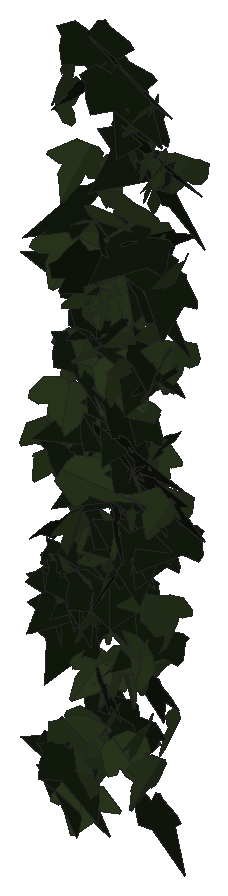
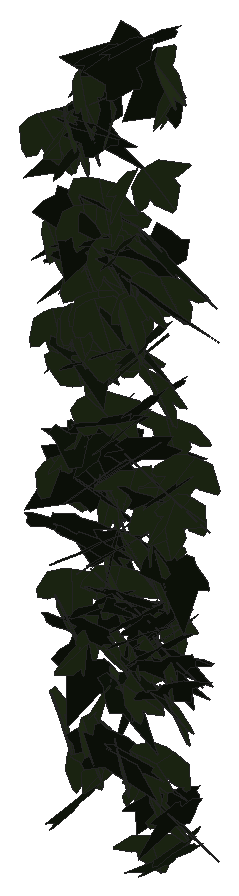
# SketchUp Ruby script. Lengths in inches.
U = 1.inch
M = Sketchup.active_model
def pt(a) = Geom::Point3d.new(a.map { |v| v * U })
def face(e, loops, mat)
  f = e.add_face(loops[0].map { |a| pt(a) })
  loops[1..].each { |l| e.add_face(l.map { |a| pt(a) }).erase! }
  f.material = f.back_material = mat if mat
  f
end
# faces: each face lists its corners as indices into pts; further lists are holes
def faces(e, pts, list, mat = nil) = list.each { |f| face(e, (f[0].is_a?(Array) ? f : [f]).map { |l| l.map { |i| pts[i] } }, mat) }
# xy, xz, yz: faces in a plane at the given z, y or x. An outline is a flat list of corners, or four numbers for a rectangle; further outlines are holes
def ring(l) = l.size == 4 ? [[l[0], l[1]], [l[2], l[1]], [l[2], l[3]], [l[0], l[3]]] : l.each_slice(2).to_a
def flat(e, list, mat, &to3) = list.each { |f| face(e, (f[0].is_a?(Array) ? f : [f]).map { |l| ring(l).map { |u, v| to3.(u, v) } }, mat) }
def xy(e, z, list, mat = nil) = flat(e, list, mat) { |x, y| [x, y, z] }
def xz(e, y, list, mat = nil) = flat(e, list, mat) { |x, z| [x, y, z] }
def yz(e, x, list, mat = nil) = flat(e, list, mat) { |y, z| [x, y, z] }
def lines(e, pts, list) = list.each { |a, b| e.add_line(pt(pts[a]), pt(pts[b])) }
# prism: a flat outline (further loops are holes) pulled along v
def prism(e, loops, v, mat = nil)
  f = face(e, loops, mat); d = Geom::Vector3d.new(v.map { |x| x * U })
  f.pushpull(f.normal.samedirection?(d) ? d.length : -d.length)
end
def box(e, o, s, mat = nil) = prism(e, [[o, [o[0] + s[0], o[1], o[2]], [o[0] + s[0], o[1] + s[1], o[2]], [o[0], o[1] + s[1], o[2]]]], [0, 0, s[2]], mat)
def at(x, y, z, deg = 0) = Geom::Transformation.translation(pt([x, y, z])) * Geom::Transformation.rotation(ORIGIN, Z_AXIS, deg.degrees)
def axes(o, x, y, z) = Geom::Transformation.new([*x, 0, *y, 0, *z, 0, *pt(o).to_a, 1])
def part(name) = M.definitions.add(name)
# library, detail: a bought-in or finely detailed component or shape, given as its bounding box
def library(name, o, s) = part(name).tap { |d| box(d.entities, o, s) }
def detail(e, o, s) = box(e.add_group.entities, o, s)
def put(e, d, t, mat = nil) = e.add_instance(d, t).tap { |i| i.material = mat if mat }
def group(e, t, mat = nil) = e.add_group.tap { |g| g.transformation = t; g.material = mat if mat }.entities
root = M.entities
M.materials.add("1026 AP 7946 SUNNY SIDE UP").color = [254, 231, 186]
M.materials.add("efeu1").color = [18, 25, 13]
M.materials.add("efeu2").color = [43, 57, 29]
c1 = part("ivyleaf_9")
p = [[1.54,2.16,1.25],[1.36,2.04,1.19],[-0.21,0.99,0.68],[-0.71,1.11,0.82],[-0.85,0.86,0.67],[-0.8,0.17,0.21],
  [-0.9,-0.01,0.1],[-0.67,-0.16,-0.02],[-0.08,-0.08,-0.05],[-0.03,-0.6,-0.4],[0.65,-0.88,-0.66],[0.83,-0.6,-0.49],
  [1.29,-0.42,-0.43],[1.8125,-0.07,-0.26],[1.21,0.44,0.15]]
faces(c1.entities,p,[[0,1,2,3,4,5,6,7,8,9,10,11,12,13,14]],"efeu1")
c2 = part("ivyleaf_10")
p = [[0,0.5,-0.03],[-0.0625,2.02,-0.43],[-0.19,2.01,-0.46],[-0.54,1.05,-0.29],[-0.52,0.625,-0.18],[-0.83,0.76,-0.28],
  [-1.16,0.64,-0.33],[-1.15,0.33,-0.24],[-0.77,-0.39,0.02],[-0.3,-0.51,0.16],[0.04,-0.48,0.23],[-0.02,2.01,-0.4375],
  [-0.06,2.01,-0.43],[0.04,-0.49,0.23],[0.67,-0.49,0.14],[1.38,0.36,-0.2],[1.375,0.51,-0.24],[0.81,0.65,-0.19],
  [0.62,0.59,-0.15],[0.6,1.09,-0.28],[0.5,1.23,-0.31]]
faces(c2.entities,p,[[0,1,2,3,4,5,6,7,8,9,10],[11,12,0,13,14,15,16,17,18,19,20]],"efeu2")
put(root,c1,axes([120.77,212.53,268.47],[-0.21091,0.19544,0.14117],[-0.17036,0.08881,-0.24117],[-0.33331,-0.16906,0.03393]),"1026 AP 7946 SUNNY SIDE UP")
put(root,c1,axes([120.59,212.47,271.88],[0.03047,0.27622,-0.0017],[0.01454,-0.00388,-0.28511],[-0.43411,0.01926,-0.00967]),"1026 AP 7946 SUNNY SIDE UP")
put(root,c2,axes([120.49,212.69,270.06],[0.30892,-0.18725,0.0155],[-0.00122,-0.02411,-0.27913],[0.29552,0.19564,-0.01735]),"1026 AP 7946 SUNNY SIDE UP")
put(root,c2,axes([120.4,212.55,272.75],[-0.1299,-0.2003,-0.193],[0.20416,0.14247,-0.21639],[0.37847,-0.1456,0.05049]),"1026 AP 7946 SUNNY SIDE UP")
put(root,c1,axes([120.51,212.87,270.33],[-0.22787,-0.21754,0.05698],[-0.02154,-0.05861,-0.26879],[0.35277,-0.1441,0.02039]),"1026 AP 7946 SUNNY SIDE UP")
put(root,c1,axes([120.47,212.9,270.74],[-0.21926,-0.23495,-0.01553],[0.03784,0.00165,-0.28071],[0.36813,-0.14011,0.0196]),"1026 AP 7946 SUNNY SIDE UP")
put(root,c1,axes([120.75,212.77,276.4],[-0.38855,0.15901,-0.04009],[0.01893,-0.05423,-0.30039],[-0.25705,-0.24435,0.03848]),"1026 AP 7946 SUNNY SIDE UP")
put(root,c2,axes([120.6,212.78,272.69],[-0.32347,-0.18709,0.05466],[-0.01134,-0.07134,-0.28276],[0.30603,-0.2004,0.04729]),"1026 AP 7946 SUNNY SIDE UP")
put(root,c1,axes([120.43,212.61,268.57],[0.11729,-0.16743,-0.2077],[-0.11802,0.18616,-0.18767],[0.39362,0.10571,0.00562]),"1026 AP 7946 SUNNY SIDE UP")
put(root,c2,axes([120.43,212.44,273.25],[-0.23849,-0.20015,-0.14493],[0.20269,0.07377,-0.25292],[0.32574,-0.19245,0.05127]),"1026 AP 7946 SUNNY SIDE UP")
put(root,c1,axes([120.66,212.76,270.72],[-0.39276,-0.10828,0.02326],[-0.01902,-0.03022,-0.27965],[0.17308,-0.24903,0.02206]),"1026 AP 7946 SUNNY SIDE UP")
put(root,c2,axes([120.73,212.49,271.13],[-0.38516,0.06364,0.1045],[-0.16887,-0.01643,-0.25757],[-0.08219,-0.26447,0.03951]),"1026 AP 7946 SUNNY SIDE UP")
put(root,c1,axes([120.45,212.84,271.07],[0.00272,-0.26809,0.06368],[0.01081,-0.06327,-0.27649],[0.43302,0.00326,0.0065]),"1026 AP 7946 SUNNY SIDE UP")
put(root,c2,axes([120.65,212.66,270.68],[0.24779,-0.22318,-0.08051],[-0.02465,0.08235,-0.27887],[0.37036,0.1548,0.03531]),"1026 AP 7946 SUNNY SIDE UP")
put(root,c1,axes([120.53,212.92,270.91],[-0.08088,-0.26218,0.05791],[-0.00108,-0.05862,-0.27539],[0.42212,-0.05039,0.01039]),"1026 AP 7946 SUNNY SIDE UP")
put(root,c2,axes([120.62,212.65,275.84],[0.4535,0.04584,-0.05555],[-0.07629,-0.03814,-0.29953],[-0.08145,0.29097,-0.02874]),"1026 AP 7946 SUNNY SIDE UP")
put(root,c1,axes([121,212.61,275.57],[-0.25442,0.17797,0.17479],[-0.25808,0.07149,-0.23952],[-0.2864,-0.22252,0.06057]),"1026 AP 7946 SUNNY SIDE UP")
put(root,c1,axes([120.41,212.74,267.96],[0.15637,-0.24977,-0.04573],[0.07062,0.06279,-0.26859],[0.3922,0.08828,0.06659]),"1026 AP 7946 SUNNY SIDE UP")
put(root,c1,axes([120.96,212.71,273.1875],[-0.35977,0.17214,0.0592],[-0.08992,0.01772,-0.29416],[-0.27031,-0.235,0.01906]),"1026 AP 7946 SUNNY SIDE UP")
put(root,c1,axes([120.51,212.67,267.97],[0.02372,-0.25998,0.09001],[0.02785,-0.08787,-0.26851],[0.4311,0.01998,0.01239]),"1026 AP 7946 SUNNY SIDE UP")
put(root,c1,axes([120.53,212.59,273],[0.18098,-0.20378,-0.17155],[-0.06162,0.1652,-0.23686],[0.40803,0.11533,0.04032]),"1026 AP 7946 SUNNY SIDE UP")
put(root,c2,axes([120.81,212.27,278.24],[-0.01673,0.04441,0.32192],[-0.20615,0.28351,-0.04448],[-0.45102,-0.13124,0.00839]),"1026 AP 7946 SUNNY SIDE UP")
put(root,c1,axes([120.9,212.65,270.92],[-0.38523,0.11048,-0.05839],[0.06896,-0.04178,-0.27637],[-0.18314,-0.24812,0.01876]),"1026 AP 7946 SUNNY SIDE UP")
put(root,c2,axes([120.67,212.48,273.79],[0.45062,0.04609,0.00801],[0.01858,-0.02635,-0.2978],[-0.07104,0.28546,-0.02705]),"1026 AP 7946 SUNNY SIDE UP")
put(root,c2,axes([120.72,212.54,278.72],[0.17726,-0.24694,0.16097],[0.08061,-0.14969,-0.28019],[0.45357,0.12311,-0.01311]),"1026 AP 7946 SUNNY SIDE UP")
put(root,c2,axes([120.9,212.59,271.83],[0.22083,-0.13823,-0.20266],[-0.16319,0.16966,-0.19895],[0.33991,0.17126,0.03615]),"1026 AP 7946 SUNNY SIDE UP")
put(root,c2,axes([120.78,212.63,274.43],[0.38706,-0.14999,-0.02647],[-0.03897,0.00706,-0.29683],[0.23586,0.24731,-0.00561]),"1026 AP 7946 SUNNY SIDE UP")
put(root,c1,axes([120.82,212.48,270.36],[-0.39867,-0.04101,-0.11302],[0.17571,-0.00821,-0.26349],[0.054,-0.27604,0.02297]),"1026 AP 7946 SUNNY SIDE UP")
put(root,c2,axes([120.8,212.52,271.97],[0.00337,-0.27731,0.01631],[0.028,-0.01724,-0.28522],[0.43601,0.00325,0.01819]),"1026 AP 7946 SUNNY SIDE UP")
put(root,c2,axes([120.8125,212.67,277.25],[-0.14321,-0.23981,0.17772],[0.04949,-0.18871,-0.25225],[0.46313,-0.05399,0.08191]),"1026 AP 7946 SUNNY SIDE UP")
put(root,c2,axes([121.11,212.34,268.38],[-0.15765,0.06453,0.26715],[-0.40903,0.03815,-0.11333],[-0.09372,-0.27505,0.04523]),"1026 AP 7946 SUNNY SIDE UP")
put(root,c1,axes([120.6875,212.76,271.2],[0.0412,-0.23113,-0.15049],[-0.04404,0.14239,-0.23858],[0.42657,0.03702,-0.01009]),"1026 AP 7946 SUNNY SIDE UP")
put(root,c1,axes([120.65,212.77,274.34],[0.06836,-0.28675,-0.05325],[-0.01159,0.04952,-0.29849],[0.45755,0.04409,0.00039]),"1026 AP 7946 SUNNY SIDE UP")
put(root,c1,axes([121.05,212.74,270.41],[-0.31423,0.17946,-0.01745],[0.00395,-0.02404,-0.27634],[-0.28357,-0.1992,0.01549]),"1026 AP 7946 SUNNY SIDE UP")
put(root,c1,axes([120.6875,212.59,271.02],[0.05028,-0.28435,-0.00671],[-0.01306,0.004,-0.29465],[0.44699,0.0321,-0.00786]),"1026 AP 7946 SUNNY SIDE UP")
put(root,c2,axes([120.92,212.87,270.16],[0.04349,-0.19285,0.19118],[0.01658,-0.18673,-0.20144],[0.42169,0.02723,-0.0118]),"1026 AP 7946 SUNNY SIDE UP")
put(root,c1,axes([120.8,212.91,271.27],[-0.06988,-0.26636,0.0551],[-0.00034,-0.05569,-0.27838],[0.42766,-0.04357,0.00878]),"1026 AP 7946 SUNNY SIDE UP")
put(root,c1,axes([121.13,212.74,273.4],[-0.30637,-0.10451,0.18234],[-0.22897,-0.1031,-0.22769],[0.22925,-0.24264,0.01627]),"1026 AP 7946 SUNNY SIDE UP")
put(root,c1,axes([120.89,212.92,270.93],[-0.17536,-0.2308,0.09651],[0.00025,-0.1041,-0.26101],[0.39245,-0.10306,0.04329]),"1026 AP 7946 SUNNY SIDE UP")
put(root,c1,axes([120.91,212.26,278.36],[0.13016,0.19676,0.2412],[0.1452,0.21394,-0.21865],[-0.45703,0.12401,-0.00077]),"1026 AP 7946 SUNNY SIDE UP")
put(root,c1,axes([120.81,212.42,268.54],[-0.02548,-0.2579,-0.1362],[0.00554,0.13077,-0.26541],[0.45462,-0.01605,-0.0044]),"1026 AP 7946 SUNNY SIDE UP")
put(root,c2,axes([120.9,212.54,267.93],[0.31945,0.1633,-0.05189],[-0.03836,-0.05118,-0.26767],[-0.26639,0.20319,-0.02369]),"1026 AP 7946 SUNNY SIDE UP")
put(root,c2,axes([121.01,212.58,268.95],[0.37013,-0.12697,-0.07378],[-0.06499,0.07091,-0.2718],[0.21923,0.23539,0.04399]),"1026 AP 7946 SUNNY SIDE UP")
put(root,c1,axes([120.82,212.84,274.85],[0.08722,-0.28821,0.02537],[-0.00204,-0.02699,-0.30245],[0.45506,0.05512,-0.00622]),"1026 AP 7946 SUNNY SIDE UP")
put(root,c2,axes([121.05,212.83,275.35],[0.06234,-0.2942,0.01418],[0.00092,-0.0155,-0.3059],[0.46323,0.03962,-0.0013]),"1026 AP 7946 SUNNY SIDE UP")
put(root,c2,axes([120.99,212.79,270.93],[0.35565,-0.14518,0.01561],[0.00311,-0.0264,-0.27618],[0.22963,0.22521,-0.02043]),"1026 AP 7946 SUNNY SIDE UP")
put(root,c1,axes([120.8125,212.77,274.99],[0.17252,-0.27635,-0.02188],[-0.0069,0.01942,-0.30618],[0.43558,0.10976,0.00381]),"1026 AP 7946 SUNNY SIDE UP")
put(root,c2,axes([120.89,212.34,268.99],[-0.31921,-0.07509,-0.16158],[0.25004,0.0158,-0.22034],[0.10915,-0.25579,0.03219]),"1026 AP 7946 SUNNY SIDE UP")
put(root,c1,axes([121.3,212.74,269.1],[-0.40247,0.05445,0.06141],[-0.0979,-0.00854,-0.26879],[-0.08027,-0.2626,0.01987]),"1026 AP 7946 SUNNY SIDE UP")
put(root,c1,axes([121.26,212.92,271.44],[-0.41632,-0.03662,0.06131],[-0.07296,-0.08327,-0.26499],[0.08253,-0.25833,0.07503]),"1026 AP 7946 SUNNY SIDE UP")
put(root,c2,axes([121.02,212.88,270.69],[-0.28806,0.12773,-0.1531],[0.05058,-0.18192,-0.20201],[-0.30483,-0.15089,0.11115]),"1026 AP 7946 SUNNY SIDE UP")
put(root,c2,axes([121.11,212.58,275.38],[-0.17996,-0.27032,-0.02899],[0.06642,0.0108,-0.30025],[0.4219,-0.117,0.0349]),"1026 AP 7946 SUNNY SIDE UP")
put(root,c2,axes([121.14,212.375,270.75],[0.00499,-0.193,-0.22209],[0.02288,0.21434,-0.19721],[0.45312,-0.0087,0.0124]),"1026 AP 7946 SUNNY SIDE UP")
put(root,c1,axes([120.96,212.15,275.74],[0.05152,0.06477,0.31651],[0.37053,0.19851,-0.06792],[-0.32542,0.23629,-0.02723]),"1026 AP 7946 SUNNY SIDE UP")
put(root,c1,axes([121.33,212.72,272.7],[-0.4221,-0.07614,0.06048],[-0.07745,-0.04212,-0.28641],[0.13032,-0.27164,0.0257]),"1026 AP 7946 SUNNY SIDE UP")
put(root,c2,axes([121.07,212.74,273.04],[0.14746,0.26906,0.01251],[0.00736,0.00961,-0.29348],[-0.42333,0.09389,-0.00075]),"1026 AP 7946 SUNNY SIDE UP")
put(root,c2,axes([121.24,212.55,271.97],[0.33831,-0.15625,-0.09999],[-0.13749,0.04297,-0.27321],[0.25363,0.23172,-0.01473]),"1026 AP 7946 SUNNY SIDE UP")
put(root,c1,axes([121.4,212.67,275.09],[-0.34323,0.20266,-0.0309],[0.01109,-0.03804,-0.30616],[-0.32221,-0.21719,0.02237]),"1026 AP 7946 SUNNY SIDE UP")
put(root,c2,axes([121.46,212.55,276.375],[0.21129,-0.03099,-0.27004],[-0.38596,0.09294,-0.1405],[0.15185,0.27935,0.01863]),"1026 AP 7946 SUNNY SIDE UP")
put(root,c1,axes([120.99,212.6,279.11],[0.04256,-0.29143,-0.11671],[0.03646,0.11363,-0.29912],[0.48936,0.01688,0.03244]),"1026 AP 7946 SUNNY SIDE UP")
put(root,c1,axes([121.42,212.81,271.48],[-0.39046,0.11841,-0.00744],[-0.00672,-0.02722,-0.28227],[-0.18648,-0.24695,0.02575]),"1026 AP 7946 SUNNY SIDE UP")
put(root,c2,axes([121.23,212.49,269.98],[0.21279,0.16933,-0.18791],[-0.14972,-0.15778,-0.22342],[-0.36277,0.16444,-0.01801]),"1026 AP 7946 SUNNY SIDE UP")
put(root,c2,axes([121.03,212.63,275.52],[0.37753,-0.09209,0.14559],[0.19266,-0.07505,-0.2643],[0.18328,0.26857,-0.02206]),"1026 AP 7946 SUNNY SIDE UP")
put(root,c1,axes([121.37,212.6,269.96],[-0.17619,0.23748,-0.0602],[0.03304,-0.05618,-0.2708],[-0.38364,-0.1139,0.00433]),"1026 AP 7946 SUNNY SIDE UP")
put(root,c2,axes([121.19,212.64,277.1],[-0.07424,0.28115,0.08679],[-0.02934,0.08066,-0.29318],[-0.45986,-0.05053,0.0047]),"1026 AP 7946 SUNNY SIDE UP")
put(root,c2,axes([121.24,212.75,269.18],[0.12519,-0.25358,-0.03744],[0.00053,0.03666,-0.27335],[0.40249,0.07883,0.01201]),"1026 AP 7946 SUNNY SIDE UP")
put(root,c1,axes([121.04,212.76,273.29],[0.11711,-0.26907,-0.06063],[0.00671,0.06051,-0.28653],[0.43252,0.07192,0.02086]),"1026 AP 7946 SUNNY SIDE UP")
put(root,c1,axes([121.23,212.47,269.86],[0.26019,-0.14062,-0.19291],[-0.26325,0.0879,-0.22084],[0.25603,0.23328,-0.03102]),"1026 AP 7946 SUNNY SIDE UP")
put(root,c2,axes([121.2,212.58,268.58],[-0.1473,0.09544,0.26007],[0.15317,-0.23665,0.1283],[0.3949,0.12738,0.04724]),"1026 AP 7946 SUNNY SIDE UP")
put(root,c2,axes([120.98,212.33,272.74],[-0.12863,-0.08934,-0.27318],[0.42213,0.05105,-0.10294],[0.12135,-0.27227,0.06851]),"1026 AP 7946 SUNNY SIDE UP")
put(root,c2,axes([121.51,212.72,274.625],[0.08493,0.09144,-0.28205],[-0.34026,-0.17229,-0.10407],[-0.30154,0.22017,0.038]),"1026 AP 7946 SUNNY SIDE UP")
put(root,c1,axes([121.125,212.81,273.7],[0.09763,-0.284,0.01254],[0.00129,-0.01393,-0.29956],[0.44709,0.06206,-0.00187]),"1026 AP 7946 SUNNY SIDE UP")
put(root,c2,axes([121.33,212.6875,271.52],[-0.3325,-0.17075,-0.04306],[0.09764,-0.01296,-0.27557],[0.25821,-0.21498,0.04876]),"1026 AP 7946 SUNNY SIDE UP")
put(root,c1,axes([121.62,212.74,269.2],[0.05554,0.02659,-0.27389],[-0.35562,-0.14011,-0.04618],[-0.22416,0.22887,0.00541]),"1026 AP 7946 SUNNY SIDE UP")
put(root,c2,axes([121.29,212.76,275.95],[0.45136,0.08506,-0.01514],[-0.00965,-0.03246,-0.30713],[-0.13551,0.28561,-0.02855]),"1026 AP 7946 SUNNY SIDE UP")
put(root,c1,axes([121.17,212.58,271.11],[-0.03876,-0.25614,-0.14899],[0.10206,0.13536,-0.2602],[0.44998,-0.05276,0.04618]),"1026 AP 7946 SUNNY SIDE UP")
put(root,c1,axes([121.57,212.82,272.68],[-0.43044,0.06295,-0.0267],[0.02795,-0.0391,-0.28748],[-0.10356,-0.27221,0.0334]),"1026 AP 7946 SUNNY SIDE UP")
put(root,c1,axes([121.41,212.28,271.14],[0.06595,0.12303,0.27274],[0.12409,0.252,-0.1324],[-0.44092,0.08932,0.00353]),"1026 AP 7946 SUNNY SIDE UP")
put(root,c2,axes([121.61,212.74,273.82],[-0.26604,-0.13233,0.19303],[-0.19837,-0.14189,-0.22054],[0.30241,-0.20949,0.02516]),"1026 AP 7946 SUNNY SIDE UP")
put(root,c2,axes([121.4,212.79,272.77],[0.26086,-0.23153,0.02971],[0.00706,-0.03382,-0.29316],[0.36706,0.16519,-0.01547]),"1026 AP 7946 SUNNY SIDE UP")
put(root,c1,axes([121.03,212.77,278.78],[0.33758,-0.19204,0.14807],[0.16756,-0.09808,-0.29732],[0.33906,0.23968,-0.00049]),"1026 AP 7946 SUNNY SIDE UP")
put(root,c1,axes([121.48,212.48,272.1875],[0.16256,-0.05061,-0.27937],[-0.35911,0.14618,-0.11708],[0.24251,0.2504,0.0139]),"1026 AP 7946 SUNNY SIDE UP")
put(root,c2,axes([121.44,212.87,276.06],[-0.0315,-0.24745,0.16942],[0.0308,-0.16697,-0.25517],[0.4674,-0.00568,0.02823]),"1026 AP 7946 SUNNY SIDE UP")
put(root,c1,axes([121.23,212.71,272],[0.13641,-0.26105,-0.09403],[0.01545,0.09698,-0.28012],[0.43381,0.07863,0.03954]),"1026 AP 7946 SUNNY SIDE UP")
put(root,c2,axes([121.48,212.49,269.91],[0.23216,-0.22512,-0.01253],[-0.02727,0.00162,-0.27698],[0.35334,0.14804,-0.01314]),"1026 AP 7946 SUNNY SIDE UP")
put(root,c2,axes([121.46,212.6,271.59],[0.09579,-0.26015,0.11821],[0.04271,-0.11301,-0.27591],[0.44598,0.0667,0.00103]),"1026 AP 7946 SUNNY SIDE UP")
put(root,c2,axes([121.46,212.73,272.63],[-0.32794,0.17699,-0.08192],[0.0177,-0.1069,-0.27271],[-0.30524,-0.19635,0.0722]),"1026 AP 7946 SUNNY SIDE UP")
put(root,c2,axes([121.55,212.77,275.18],[-0.23229,-0.24808,0.06185],[-0.00644,-0.06866,-0.29614],[0.40181,-0.14452,0.03101]),"1026 AP 7946 SUNNY SIDE UP")
put(root,c2,axes([121.45,212.78,269.9375],[-0.0801,0.25628,-0.06404],[0.00698,-0.06396,-0.26943],[-0.41514,-0.05053,0.00783]),"1026 AP 7946 SUNNY SIDE UP")
put(root,c1,axes([121.52,212.8,273.66],[-0.26233,-0.23031,0.05312],[-0.01171,-0.05956,-0.29186],[0.37138,-0.16457,0.02832]),"1026 AP 7946 SUNNY SIDE UP")
put(root,c1,axes([121.68,212.45,276.31],[-0.06775,0.29914,0.01302],[-0.00281,0.0108,-0.31129],[-0.47068,-0.04312,-0.00002]),"1026 AP 7946 SUNNY SIDE UP")
put(root,c2,axes([121.67,212.63,276.74],[-0.44531,0.0265,0.09813],[-0.15262,-0.0219,-0.2916],[-0.02838,-0.29794,0.0284]),"1026 AP 7946 SUNNY SIDE UP")
put(root,c2,axes([121.57,212.73,275.26],[-0.28816,-0.23661,0.03067],[0.03561,-0.05629,-0.30394],[0.37355,-0.17715,0.05263]),"1026 AP 7946 SUNNY SIDE UP")
put(root,c1,axes([121.3,212.73,276.1],[0.1608,-0.27928,0.05977],[0.0254,-0.05755,-0.30669],[0.44831,0.10343,-0.00407]),"1026 AP 7946 SUNNY SIDE UP")
put(root,c2,axes([121.51,212.64,277.85],[-0.24317,0.25825,-0.02177],[0.0027,-0.02529,-0.31003],[-0.40762,-0.15423,0.01093]),"1026 AP 7946 SUNNY SIDE UP")
put(root,c1,axes([121.53,212.87,271.16],[-0.17888,-0.22869,0.09326],[-0.04957,-0.0868,-0.26345],[0.38432,-0.11764,0.00943]),"1026 AP 7946 SUNNY SIDE UP")
put(root,c1,axes([121.42,212.67,273.73],[0.18492,-0.25029,-0.09156],[-0.0831,0.07162,-0.28396],[0.40852,0.12786,-0.01632]),"1026 AP 7946 SUNNY SIDE UP")
put(root,c2,axes([121.47,212.52,274.42],[0.21625,0.24014,0.12269],[0.10748,0.09643,-0.28432],[-0.40656,0.15322,-0.0099]),"1026 AP 7946 SUNNY SIDE UP")
put(root,c2,axes([121.68,212.25,274.47],[0.04652,0.20067,0.21945],[-0.14903,0.20802,-0.18812],[-0.43399,-0.04993,0.08812]),"1026 AP 7946 SUNNY SIDE UP")
put(root,c1,axes([121.58,212.89,278.12],[-0.1842,-0.24211,0.14833],[-0.00042,-0.15727,-0.271],[0.44403,-0.10058,0.06127]),"1026 AP 7946 SUNNY SIDE UP")
put(root,c1,axes([121.46,212.48,278.72],[0.06961,-0.25385,-0.20476],[-0.0076,0.19863,-0.26322],[0.50551,0.03794,0.02424]),"1026 AP 7946 SUNNY SIDE UP")
put(root,c1,axes([121.85,212.75,277.64],[-0.46524,-0.04991,0.00537],[-0.00047,-0.03109,-0.30769],[0.07896,-0.29429,0.02981]),"1026 AP 7946 SUNNY SIDE UP")
put(root,c2,axes([121.73,212.77,275.62],[-0.24477,-0.24167,0.08931],[0.00696,-0.10544,-0.29064],[0.40439,-0.14446,0.05906]),"1026 AP 7946 SUNNY SIDE UP")
put(root,c1,axes([121.79,212.83,272],[-0.42191,-0.06805,-0.05354],[0.09556,-0.0327,-0.28142],[0.09432,-0.27127,0.04565]),"1026 AP 7946 SUNNY SIDE UP")
put(root,c2,axes([121.57,212.49,268.84],[0.16833,0.23237,0.12278],[0.08177,0.1058,-0.26293],[-0.40144,0.11899,-0.00207]),"1026 AP 7946 SUNNY SIDE UP")
put(root,c2,axes([121.76,212.77,276.41],[-0.25263,-0.25506,0.00757],[0.03177,-0.02307,-0.3092],[0.40004,-0.15924,0.02933]),"1026 AP 7946 SUNNY SIDE UP")
put(root,c1,axes([121.54,212.73,272.87],[0.13737,-0.2629,-0.06679],[-0.01143,0.06425,-0.28471],[0.42505,0.08669,0.01393]),"1026 AP 7946 SUNNY SIDE UP")
put(root,c1,axes([121.68,212.83,274.49],[-0.18029,-0.25752,0.08131],[0.00387,-0.08834,-0.28845],[0.42418,-0.10865,0.03719]),"1026 AP 7946 SUNNY SIDE UP")
put(root,c1,axes([121.36,212.5625,273.1875],[0.29428,-0.11539,0.20883],[0.26058,-0.1183,-0.22695],[0.25936,0.24977,-0.00892]),"1026 AP 7946 SUNNY SIDE UP")
put(root,c1,axes([121.52,212.83,273.31],[0.22805,-0.24554,0.02258],[0.00883,-0.02375,-0.29383],[0.38773,0.14496,-0.00659]),"1026 AP 7946 SUNNY SIDE UP")
put(root,c1,axes([121.65,212.56,271.97],[-0.23194,-0.19723,-0.14658],[0.15994,0.09969,-0.2524],[0.34622,-0.17818,0.0184]),"1026 AP 7946 SUNNY SIDE UP")
put(root,c2,axes([121.82,212.72,278.22],[0.01406,-0.30675,-0.03968],[0.00724,0.03692,-0.31587],[0.48573,0.00833,0.00585]),"1026 AP 7946 SUNNY SIDE UP")
put(root,c2,axes([121.99,212.33,270.43],[0.24832,-0.11804,-0.22182],[-0.28868,0.11204,-0.20197],[0.255,0.24178,-0.01265]),"1026 AP 7946 SUNNY SIDE UP")
put(root,c1,axes([121.95,212.55,276.48],[-0.47173,-0.03086,-0.03216],[0.05525,-0.04155,-0.30751],[0.04104,-0.29873,0.0443]),"1026 AP 7946 SUNNY SIDE UP")
put(root,c1,axes([122,212.54,274.375],[0.00142,0.26,0.13959],[-0.13603,0.12826,-0.25499],[-0.43936,-0.03887,0.0794]),"1026 AP 7946 SUNNY SIDE UP")
put(root,c1,axes([122,212.75,273.28],[-0.23787,0.22816,-0.0771],[0.00855,-0.08667,-0.27923],[-0.37811,-0.14549,0.04219]),"1026 AP 7946 SUNNY SIDE UP")
put(root,c2,axes([121.85,212.6,269.17],[0.04588,-0.2792,-0.02343],[-0.01923,0.01998,-0.28889],[0.43985,0.02999,-0.01019]),"1026 AP 7946 SUNNY SIDE UP")
put(root,c1,axes([121.76,212.92,271.82],[-0.14523,-0.23689,0.11243],[-0.00256,-0.11665,-0.25976],[0.411,-0.08443,0.03811]),"1026 AP 7946 SUNNY SIDE UP")
put(root,c2,axes([121.89,212.79,274.99],[-0.05919,-0.29503,0.00534],[0.00055,-0.00696,-0.30644],[0.46402,-0.03763,0.00105]),"1026 AP 7946 SUNNY SIDE UP")
put(root,c2,axes([121.93,212.59,277.81],[0.20024,-0.25115,-0.13375],[-0.09079,0.11469,-0.28942],[0.43413,0.13982,0.00117]),"1026 AP 7946 SUNNY SIDE UP")
put(root,c1,axes([121.82,212.83,276],[-0.20148,-0.26969,0.03862],[-0.00619,-0.04128,-0.3075],[0.42844,-0.12742,0.01372]),"1026 AP 7946 SUNNY SIDE UP")
put(root,c1,axes([121.87,212.61,276.36],[0.21087,0.26478,0.01628],[0.03477,0.0048,-0.30521],[-0.4155,0.13478,-0.01728]),"1026 AP 7946 SUNNY SIDE UP")
put(root,c1,axes([121.54,212.66,277.76],[0.36869,-0.13854,0.13438],[0.17406,-0.07059,-0.28095],[0.2444,0.25926,-0.00263]),"1026 AP 7946 SUNNY SIDE UP")
put(root,c1,axes([121.89,212.51,270.0625],[0.38826,-0.02904,-0.152],[-0.2342,-0.01052,-0.255],[0.03066,0.28737,-0.02299]),"1026 AP 7946 SUNNY SIDE UP")
put(root,c1,axes([122.09,212.7,270.66],[-0.40756,-0.07746,0.00566],[0.00235,-0.02562,-0.27765],[0.12214,-0.258,0.02421]),"1026 AP 7946 SUNNY SIDE UP")
put(root,c1,axes([121.87,212.47,274.87],[0.26668,-0.14313,-0.2123],[-0.18801,0.17147,-0.22395],[0.34565,0.2037,0.04197]),"1026 AP 7946 SUNNY SIDE UP")
put(root,c2,axes([121.93,212.82,273.2],[0.00914,0.26636,-0.11227],[0.00258,-0.11054,-0.27509],[-0.45343,0.00474,-0.00383]),"1026 AP 7946 SUNNY SIDE UP")
put(root,c2,axes([121.99,212.43,270.22],[-0.00794,-0.06902,-0.30429],[0.11468,0.28606,-0.06857],[0.46234,-0.07214,0.01178]),"1026 AP 7946 SUNNY SIDE UP")
put(root,c2,axes([122.04,212.56,268.69],[-0.01823,-0.23281,0.1791],[0.04722,-0.17533,-0.23903],[0.45568,0.00886,0.03194]),"1026 AP 7946 SUNNY SIDE UP")
put(root,c2,axes([121.96,212.75,274.22],[-0.00007,-0.32774,-0.07006],[0.0218,-0.06609,0.33695],[-0.52527,-0.0027,0.01399]),"1026 AP 7946 SUNNY SIDE UP")
put(root,c2,axes([122.1,212.61,277.56],[0.11796,-0.29954,-0.02425],[-0.02847,0.01796,-0.31772],[0.47139,0.07604,-0.01312]),"1026 AP 7946 SUNNY SIDE UP")
put(root,c1,axes([122.15,212.9,272.15],[-0.37726,-0.14503,0.01189],[0.00269,-0.02665,-0.28794],[0.22885,-0.23876,0.02299]),"1026 AP 7946 SUNNY SIDE UP")
put(root,c2,axes([122.125,212.59,271.14],[-0.3391,-0.18208,0.00022],[0.0178,-0.01534,-0.29019],[0.28575,-0.21512,0.01834]),"1026 AP 7946 SUNNY SIDE UP")
put(root,c1,axes([121.91,212.63,275.65],[0.2437,-0.23652,-0.09327],[-0.0742,0.07571,-0.29086],[0.39047,0.162,0.00293]),"1026 AP 7946 SUNNY SIDE UP")
put(root,c1,axes([121.875,212.64,272.77],[0.4478,-0.04157,-0.00065],[-0.0069,-0.02736,-0.29528],[0.065,0.28347,-0.02688]),"1026 AP 7946 SUNNY SIDE UP")
put(root,c2,axes([122.26,212.66,272.68],[-0.22041,-0.22025,0.13559],[-0.03922,-0.13896,-0.26523],[0.40256,-0.13413,0.0484]),"1026 AP 7946 SUNNY SIDE UP")
put(root,c2,axes([122.31,212.86,277.53],[-0.24109,-0.22846,0.12624],[-0.08875,-0.11108,-0.28374],[0.39886,-0.16281,0.01317]),"1026 AP 7946 SUNNY SIDE UP")
put(root,c2,axes([122.22,212.77,274.81],[-0.22865,-0.25248,0.05545],[0.03603,-0.07575,-0.29487],[0.40479,-0.13587,0.05756]),"1026 AP 7946 SUNNY SIDE UP")
put(root,c2,axes([122.17,212.46,277.39],[-0.00833,-0.06541,-0.32464],[0.08957,0.30962,-0.06546],[0.49749,-0.05684,0.00635]),"1026 AP 7946 SUNNY SIDE UP")
put(root,c1,axes([122,212.61,268.11],[0.15475,-0.27228,-0.01208],[-0.01584,0.00718,-0.29813],[0.42813,0.09868,-0.00667]),"1026 AP 7946 SUNNY SIDE UP")
put(root,c1,axes([121.97,212.73,277.3125],[0.30921,-0.23375,-0.0383],[-0.04828,0.021,-0.3144],[0.3687,0.19879,-0.00904]),"1026 AP 7946 SUNNY SIDE UP")
put(root,c2,axes([122.27,212.77,276.04],[0.04461,-0.30012,0.02535],[-0.00177,-0.02653,-0.31069],[0.47371,0.02816,-0.00355]),"1026 AP 7946 SUNNY SIDE UP")
put(root,c2,axes([122.25,212.65,270.84],[0.22601,-0.24126,0.00536],[-0.02074,-0.01549,-0.28872],[0.37894,0.14305,-0.019]),"1026 AP 7946 SUNNY SIDE UP")
put(root,c1,axes([122.14,212.69,275.92],[-0.08668,-0.28684,0.05127],[-0.00395,-0.05184,-0.30112],[0.45819,-0.05471,0.0071]),"1026 AP 7946 SUNNY SIDE UP")
put(root,c2,axes([122.31,212.63,269.39],[0.16958,-0.2567,-0.052],[-0.03532,0.04373,-0.28656],[0.40941,0.1101,-0.00318]),"1026 AP 7946 SUNNY SIDE UP")
